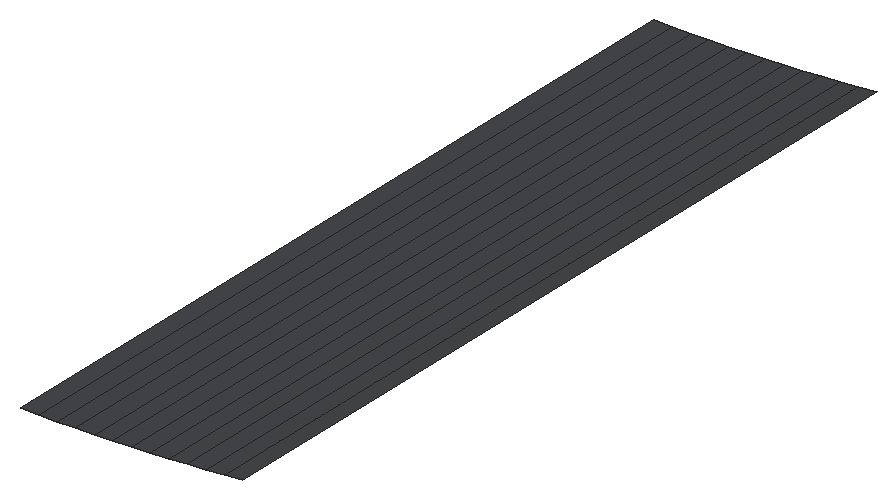
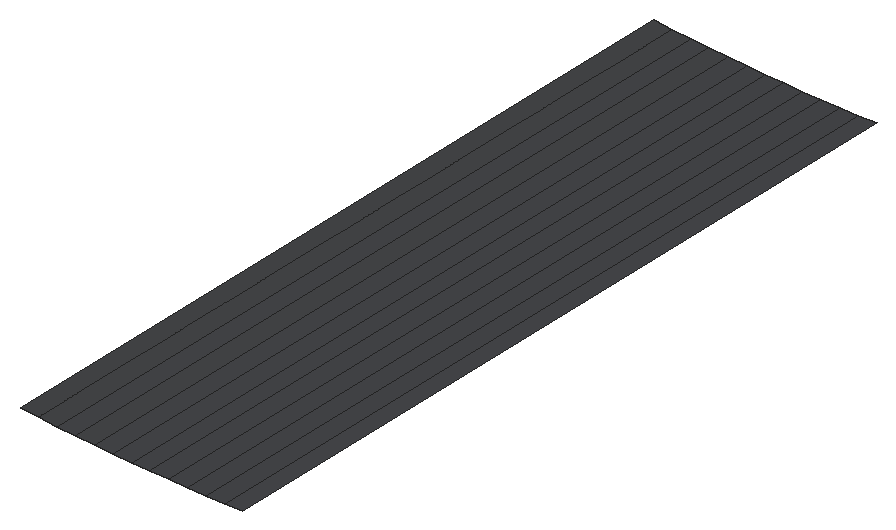
# SketchUp Ruby script. Lengths in inches.
U = 1.inch
M = Sketchup.active_model
def pt(a) = Geom::Point3d.new(a.map { |v| v * U })
def face(e, loops, mat)
  f = e.add_face(loops[0].map { |a| pt(a) })
  loops[1..].each { |l| e.add_face(l.map { |a| pt(a) }).erase! }
  f.material = f.back_material = mat if mat
  f
end
# faces: each face lists its corners as indices into pts; further lists are holes
def faces(e, pts, list, mat = nil) = list.each { |f| face(e, (f[0].is_a?(Array) ? f : [f]).map { |l| l.map { |i| pts[i] } }, mat) }
# xy, xz, yz: faces in a plane at the given z, y or x. An outline is a flat list of corners, or four numbers for a rectangle; further outlines are holes
def ring(l) = l.size == 4 ? [[l[0], l[1]], [l[2], l[1]], [l[2], l[3]], [l[0], l[3]]] : l.each_slice(2).to_a
def flat(e, list, mat, &to3) = list.each { |f| face(e, (f[0].is_a?(Array) ? f : [f]).map { |l| ring(l).map { |u, v| to3.(u, v) } }, mat) }
def xy(e, z, list, mat = nil) = flat(e, list, mat) { |x, y| [x, y, z] }
def xz(e, y, list, mat = nil) = flat(e, list, mat) { |x, z| [x, y, z] }
def yz(e, x, list, mat = nil) = flat(e, list, mat) { |y, z| [x, y, z] }
def lines(e, pts, list) = list.each { |a, b| e.add_line(pt(pts[a]), pt(pts[b])) }
# prism: a flat outline (further loops are holes) pulled along v
def prism(e, loops, v, mat = nil)
  f = face(e, loops, mat); d = Geom::Vector3d.new(v.map { |x| x * U })
  f.pushpull(f.normal.samedirection?(d) ? d.length : -d.length)
end
def box(e, o, s, mat = nil) = prism(e, [[o, [o[0] + s[0], o[1], o[2]], [o[0] + s[0], o[1] + s[1], o[2]], [o[0], o[1] + s[1], o[2]]]], [0, 0, s[2]], mat)
def at(x, y, z, deg = 0) = Geom::Transformation.translation(pt([x, y, z])) * Geom::Transformation.rotation(ORIGIN, Z_AXIS, deg.degrees)
def axes(o, x, y, z) = Geom::Transformation.new([*x, 0, *y, 0, *z, 0, *pt(o).to_a, 1])
def part(name) = M.definitions.add(name)
# library, detail: a bought-in or finely detailed component or shape, given as its bounding box
def library(name, o, s) = part(name).tap { |d| box(d.entities, o, s) }
def detail(e, o, s) = box(e.add_group.entities, o, s)
def put(e, d, t, mat = nil) = e.add_instance(d, t).tap { |i| i.material = mat if mat }
def group(e, t, mat = nil) = e.add_group.tap { |g| g.transformation = t; g.material = mat if mat }.entities
root = M.entities
M.materials.add("1432 AP 8245 TAR ROAD").color = [71, 72, 75]
xy(root,155.8,[[537.57,95.37,537.85,107.37]],"1432 AP 8245 TAR ROAD")
p = [[537.85,107.37,155.8],[538.13,107.37,155.81],[538.13,95.37,155.81],[537.85,95.37,155.8],[538.41,107.37,155.82],[538.41,95.37,155.82],
  [538.7,107.37,155.83],[538.7,95.37,155.83],[538.98,107.37,155.85],[538.98,95.37,155.85],[539.26,107.37,155.86],[539.26,95.37,155.86],
  [539.54,107.37,155.88],[539.54,95.37,155.88],[539.82,107.37,155.9],[539.82,95.37,155.9],[540.11,107.37,155.93],[540.11,95.37,155.93],
  [540.39,107.37,155.95],[540.39,95.37,155.95],[540.67,107.37,155.98],[540.67,95.37,155.98],[540.95,107.37,156.01],[540.95,95.37,156.01]]
faces(root,p,[[0,1,2,3],[1,4,5,2],[4,6,7,5],[6,8,9,7],[8,10,11,9],[10,12,13,11],[12,14,15,13],[14,16,17,15],
  [16,18,19,17],[18,20,21,19],[20,22,23,21]],"1432 AP 8245 TAR ROAD")
